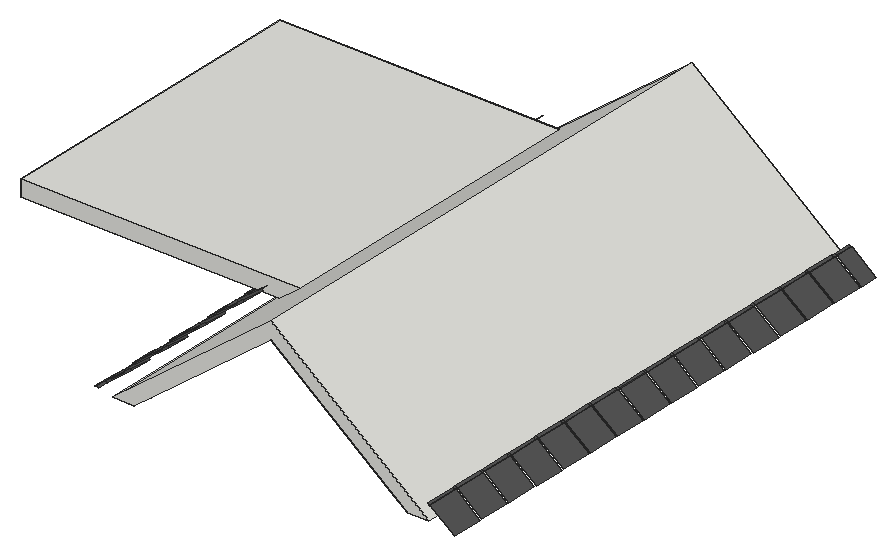
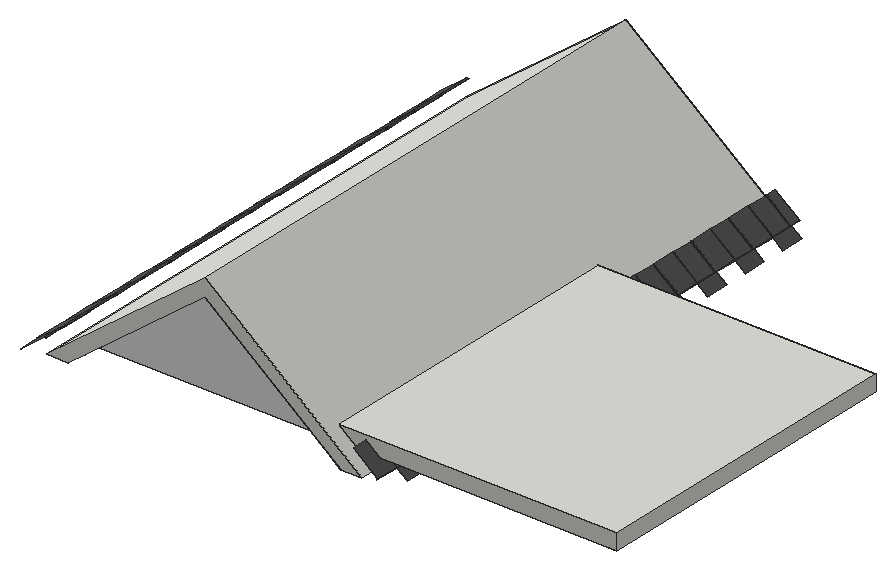
# SketchUp Ruby script. Lengths in inches.
U = 1.inch
M = Sketchup.active_model
def pt(a) = Geom::Point3d.new(a.map { |v| v * U })
def face(e, loops, mat)
  f = e.add_face(loops[0].map { |a| pt(a) })
  loops[1..].each { |l| e.add_face(l.map { |a| pt(a) }).erase! }
  f.material = f.back_material = mat if mat
  f
end
# faces: each face lists its corners as indices into pts; further lists are holes
def faces(e, pts, list, mat = nil) = list.each { |f| face(e, (f[0].is_a?(Array) ? f : [f]).map { |l| l.map { |i| pts[i] } }, mat) }
# xy, xz, yz: faces in a plane at the given z, y or x. An outline is a flat list of corners, or four numbers for a rectangle; further outlines are holes
def ring(l) = l.size == 4 ? [[l[0], l[1]], [l[2], l[1]], [l[2], l[3]], [l[0], l[3]]] : l.each_slice(2).to_a
def flat(e, list, mat, &to3) = list.each { |f| face(e, (f[0].is_a?(Array) ? f : [f]).map { |l| ring(l).map { |u, v| to3.(u, v) } }, mat) }
def xy(e, z, list, mat = nil) = flat(e, list, mat) { |x, y| [x, y, z] }
def xz(e, y, list, mat = nil) = flat(e, list, mat) { |x, z| [x, y, z] }
def yz(e, x, list, mat = nil) = flat(e, list, mat) { |y, z| [x, y, z] }
def lines(e, pts, list) = list.each { |a, b| e.add_line(pt(pts[a]), pt(pts[b])) }
# prism: a flat outline (further loops are holes) pulled along v
def prism(e, loops, v, mat = nil)
  f = face(e, loops, mat); d = Geom::Vector3d.new(v.map { |x| x * U })
  f.pushpull(f.normal.samedirection?(d) ? d.length : -d.length)
end
def box(e, o, s, mat = nil) = prism(e, [[o, [o[0] + s[0], o[1], o[2]], [o[0] + s[0], o[1] + s[1], o[2]], [o[0], o[1] + s[1], o[2]]]], [0, 0, s[2]], mat)
def at(x, y, z, deg = 0) = Geom::Transformation.translation(pt([x, y, z])) * Geom::Transformation.rotation(ORIGIN, Z_AXIS, deg.degrees)
def axes(o, x, y, z) = Geom::Transformation.new([*x, 0, *y, 0, *z, 0, *pt(o).to_a, 1])
def part(name) = M.definitions.add(name)
# library, detail: a bought-in or finely detailed component or shape, given as its bounding box
def library(name, o, s) = part(name).tap { |d| box(d.entities, o, s) }
def detail(e, o, s) = box(e.add_group.entities, o, s)
def put(e, d, t, mat = nil) = e.add_instance(d, t).tap { |i| i.material = mat if mat }
def group(e, t, mat = nil) = e.add_group.tap { |g| g.transformation = t; g.material = mat if mat }.entities
root = M.entities
M.materials.add("[Color M01]").color = [226, 226, 226]
M.materials.add("[Color M06]").color = [86, 86, 86]
xz(root,145.1875,[[245.03,334.59,244.23,335.61,263.13,350.4,263.4375,350.01,263.93,349.38]],"[Color M06]")
xz(root,163.1875,[[245.03,334.59,263.93,349.38,263.4375,350.01,263.13,350.4,244.23,335.61]],"[Color M06]")
xz(root,181.1875,[[245.03,334.59,244.54,335.22,244.23,335.61,263.13,350.4,263.4375,350.01,263.93,349.38]],"[Color M06]")
xz(root,199.1875,[[245.03,334.59,263.93,349.38,263.4375,350.01,263.13,350.4,244.23,335.61,244.54,335.22]],"[Color M06]")
xz(root,217.1875,[[245.03,334.59,244.54,335.22,244.23,335.61,263.13,350.4,263.4375,350.01,263.93,349.38]],"[Color M06]")
xz(root,235.1875,[[245.03,334.59,263.93,349.38,263.4375,350.01,263.13,350.4,244.23,335.61,244.54,335.22]],"[Color M06]")
xz(root,253.1875,[[245.03,334.59,244.23,335.61,263.13,350.4,263.4375,350.01,263.93,349.38]],"[Color M06]")
xz(root,271.1875,[[245.03,334.59,263.93,349.38,263.4375,350.01,263.13,350.4,244.23,335.61]],"[Color M06]")
xz(root,289.1875,[[245.03,334.59,244.54,335.22,244.23,335.61,263.13,350.4,263.4375,350.01,263.93,349.38]],"[Color M06]")
xz(root,307.1875,[[245.03,334.59,263.93,349.38,263.4375,350.01,263.13,350.4,244.23,335.61,244.54,335.22]],"[Color M06]")
xz(root,325.1875,[[245.03,334.59,244.54,335.22,244.23,335.61,263.13,350.4,263.4375,350.01,263.93,349.38]],"[Color M06]")
xz(root,343.1875,[[245.03,334.59,263.93,349.38,263.4375,350.01,263.13,350.4,244.23,335.61,244.54,335.22]],"[Color M06]")
xz(root,361.1875,[[245.03,334.59,244.54,335.22,244.23,335.61,263.13,350.4,263.4375,350.01,263.93,349.38]],"[Color M06]")
xz(root,379.1875,[[245.03,334.59,263.93,349.38,263.4375,350.01,263.13,350.4,244.23,335.61,244.54,335.22]],"[Color M06]")
xz(root,397.1875,[[245.03,334.59,244.23,335.61,263.13,350.4,263.4375,350.01,263.93,349.38]],"[Color M06]")
xz(root,415.1875,[[245.03,334.59,263.93,349.38,263.4375,350.01,263.13,350.4,244.23,335.61]],"[Color M06]")
xz(root,433.1875,[[245.03,334.59,244.23,335.61,263.13,350.4,263.4375,350.01,263.93,349.38]],"[Color M06]")
xz(root,451.1875,[[245.03,334.59,263.93,349.38,263.4375,350.01,263.13,350.4,244.23,335.61]],"[Color M06]")
xz(root,469.1875,[[245.03,334.59,244.54,335.22,244.23,335.61,263.13,350.4,263.4375,350.01,263.93,349.38]],"[Color M06]")
xz(root,487.1875,[[245.03,334.59,263.93,349.38,263.4375,350.01,263.13,350.4,244.23,335.61,244.54,335.22]],"[Color M06]")
xz(root,505.1875,[[245.03,334.59,244.54,335.22,244.23,335.61,263.13,350.4,263.4375,350.01,263.93,349.38]],"[Color M06]")
xz(root,523.1875,[[245.03,334.59,263.93,349.38,263.4375,350.01,263.08,350.46,244.18,335.67,244.23,335.61,244.54,335.22]],"[Color M06]")
p = [[518.42,161.375,328.98],[499.52,161.375,343.77],[499.52,137.375,343.77],[518.42,137.375,328.98],[518.42,187.375,328.98],[499.52,187.375,343.77],
  [499.52,163.375,343.77],[518.42,163.375,328.98],[518.42,213.375,328.98],[499.52,213.375,343.77],[499.52,189.375,343.77],[518.42,189.375,328.98],
  [518.42,239.375,328.98],[499.52,239.375,343.77],[499.52,215.375,343.77],[518.42,215.375,328.98],[518.42,265.375,328.98],[499.52,265.375,343.77],
  [499.52,241.375,343.77],[518.42,241.375,328.98],[518.42,291.375,328.98],[499.52,291.375,343.77],[499.52,267.375,343.77],[518.42,267.375,328.98],
  [518.42,317.375,328.98],[499.52,317.375,343.77],[499.52,293.375,343.77],[518.42,293.375,328.98],[518.42,343.375,328.98],[499.52,343.375,343.77],
  [499.52,319.375,343.77],[518.42,319.375,328.98],[518.42,369.375,328.98],[499.52,369.375,343.77],[499.52,345.375,343.77],[518.42,345.375,328.98],
  [518.42,395.375,328.98],[499.52,395.375,343.77],[499.52,371.375,343.77],[518.42,371.375,328.98],[518.42,421.375,328.98],[499.52,421.375,343.77],
  [499.52,397.375,343.77],[518.42,397.375,328.98],[518.42,447.375,328.98],[499.52,447.375,343.77],[499.52,423.375,343.77],[518.42,423.375,328.98],
  [518.42,473.375,328.98],[499.52,473.375,343.77],[499.52,449.375,343.77],[518.42,449.375,328.98],[518.42,499.375,328.98],[499.52,499.375,343.77],
  [499.52,475.375,343.77],[518.42,475.375,328.98],[518.42,525.375,328.98],[499.52,525.375,343.77],[499.52,501.375,343.77],[518.42,501.375,328.98],
  [518.42,541.1875,328.98],[499.52,541.1875,343.77],[499.52,527.375,343.77],[518.42,527.375,328.98],[236.06,145.1875,329.21],[244.23,145.1875,335.61],
  [244.23,163.1875,335.61],[236.06,163.1875,329.21],[236.06,181.1875,329.21],[244.23,181.1875,335.61],[244.23,199.1875,335.61],[236.06,199.1875,329.21],
  [236.06,217.1875,329.21],[244.23,217.1875,335.61],[244.23,235.1875,335.61],[236.06,235.1875,329.21],[236.06,253.1875,329.21],[244.23,253.1875,335.61],
  [244.23,271.1875,335.61],[236.06,271.1875,329.21],[236.06,289.1875,329.21],[244.23,289.1875,335.61],[244.23,307.1875,335.61],[236.06,307.1875,329.21],
  [236.06,325.1875,329.21],[244.23,325.1875,335.61],[244.23,343.1875,335.61],[236.06,343.1875,329.21],[236.06,361.1875,329.21],[244.23,361.1875,335.61],
  [244.23,379.1875,335.61],[236.06,379.1875,329.21],[236.06,397.1875,329.21],[244.23,397.1875,335.61],[244.23,415.1875,335.61],[236.06,415.1875,329.21],
  [236.06,433.1875,329.21],[244.23,433.1875,335.61],[244.23,451.1875,335.61],[236.06,451.1875,329.21],[236.06,469.1875,329.21],[244.23,469.1875,335.61],
  [244.23,487.1875,335.61],[236.06,487.1875,329.21],[236.06,505.1875,329.21],[244.23,505.1875,335.61],[244.23,523.1875,335.61],[236.06,523.1875,329.21],
  [245.03,145.1875,334.59],[245.03,137.375,334.59],[244.23,137.375,335.61],[245.03,163.1875,334.59],[263.93,145.1875,349.38],[263.93,163.1875,349.38],
  [245.03,181.1875,334.59],[244.54,181.1875,335.22],[245.03,199.1875,334.59],[244.54,199.1875,335.22],[263.93,181.1875,349.38],[263.93,199.1875,349.38],
  [245.03,217.1875,334.59],[244.54,217.1875,335.22],[245.03,235.1875,334.59],[244.54,235.1875,335.22],[263.93,217.1875,349.38],[263.93,235.1875,349.38],
  [245.03,253.1875,334.59],[245.03,271.1875,334.59],[263.93,253.1875,349.38],[263.93,271.1875,349.38],[245.03,289.1875,334.59],[244.54,289.1875,335.22],
  [245.03,307.1875,334.59],[244.54,307.1875,335.22],[263.93,289.1875,349.38],[263.93,307.1875,349.38],[245.03,325.1875,334.59],[244.54,325.1875,335.22],
  [245.03,343.1875,334.59],[244.54,343.1875,335.22],[263.93,325.1875,349.38],[263.93,343.1875,349.38],[245.03,361.1875,334.59],[244.54,361.1875,335.22],
  [245.03,379.1875,334.59],[244.54,379.1875,335.22],[263.93,361.1875,349.38],[263.93,379.1875,349.38],[245.03,397.1875,334.59],[245.03,415.1875,334.59],
  [263.93,397.1875,349.38],[263.93,415.1875,349.38],[245.03,433.1875,334.59],[245.03,451.1875,334.59],[263.93,433.1875,349.38],[263.93,451.1875,349.38],
  [245.03,469.1875,334.59],[244.54,469.1875,335.22],[245.03,487.1875,334.59],[244.54,487.1875,335.22],[263.93,469.1875,349.38],[263.93,487.1875,349.38],
  [245.03,505.1875,334.59],[244.54,505.1875,335.22],[245.03,523.1875,334.59],[244.54,523.1875,335.22],[263.93,505.1875,349.38],[263.93,523.1875,349.38],
  [245.03,541.1875,334.59],[244.18,523.1875,335.67],[244.18,541.1875,335.67],[263.13,137.375,350.4],[263.13,145.1875,350.4],[263.13,163.1875,350.4],
  [263.13,181.1875,350.4],[263.13,199.1875,350.4],[263.13,217.1875,350.4],[263.13,235.1875,350.4],[263.13,253.1875,350.4],[263.13,271.1875,350.4],
  [263.13,289.1875,350.4],[263.13,307.1875,350.4],[263.13,325.1875,350.4],[263.13,343.1875,350.4],[263.13,361.1875,350.4],[263.13,379.1875,350.4],
  [263.13,397.1875,350.4],[263.13,415.1875,350.4],[263.13,433.1875,350.4],[263.13,451.1875,350.4],[263.13,469.1875,350.4],[263.13,487.1875,350.4],
  [263.13,505.1875,350.4],[263.08,523.1875,350.46],[263.08,541.1875,350.46],[497.33,137.375,344.21],[498.91,137.375,342.98],[498.91,161.375,342.98],
  [497.33,161.375,344.21],[498.91,163.375,342.98],[497.33,163.375,344.21],[498.91,187.375,342.98],[497.33,187.375,344.21],[498.91,189.375,342.98],
  [497.33,189.375,344.21],[498.91,213.375,342.98],[497.33,213.375,344.21],[498.91,215.375,342.98],[497.33,215.375,344.21],[498.91,239.375,342.98],
  [497.33,239.375,344.21],[498.91,241.375,342.98],[497.33,241.375,344.21],[498.91,265.375,342.98],[497.33,265.375,344.21],[498.91,267.375,342.98],
  [497.33,267.375,344.21],[498.91,291.375,342.98],[497.33,291.375,344.21],[498.91,293.375,342.98],[497.33,293.375,344.21],[498.91,317.375,342.98],
  [497.33,317.375,344.21],[498.91,319.375,342.98],[497.33,319.375,344.21],[498.91,343.375,342.98],[497.33,343.375,344.21],[498.91,345.375,342.98],
  [497.33,345.375,344.21],[498.91,369.375,342.98],[497.33,369.375,344.21],[498.91,371.375,342.98],[497.33,371.375,344.21],[498.91,395.375,342.98],
  [497.33,395.375,344.21],[498.91,397.375,342.98],[497.33,397.375,344.21],[498.91,421.375,342.98],[497.33,421.375,344.21],[498.91,423.375,342.98],
  [497.33,423.375,344.21],[498.91,447.375,342.98],[497.33,447.375,344.21],[498.91,449.375,342.98],[497.33,449.375,344.21],[498.91,473.375,342.98],
  [497.33,473.375,344.21],[498.91,475.375,342.98],[497.33,475.375,344.21],[498.91,499.375,342.98],[497.33,499.375,344.21],[498.91,501.375,342.98],
  [497.33,501.375,344.21],[498.91,525.375,342.98],[497.33,525.375,344.21],[498.91,527.375,342.98],[497.33,527.375,344.21],[498.91,541.1875,342.98],
  [497.33,541.1875,344.21]]
faces(root,p,[[0,1,2,3],[4,5,6,7],[8,9,10,11],[12,13,14,15],[16,17,18,19],[20,21,22,23],[24,25,26,27],[28,29,30,31],
  [32,33,34,35],[36,37,38,39],[40,41,42,43],[44,45,46,47],[48,49,50,51],[52,53,54,55],[56,57,58,59],[60,61,62,63],
  [64,65,66,67],[68,69,70,71],[72,73,74,75],[76,77,78,79],[80,81,82,83],[84,85,86,87],[88,89,90,91],[92,93,94,95],
  [96,97,98,99],[100,101,102,103],[104,105,106,107],[108,109,110,65],[108,111,66,65],[108,112,113,111],[114,111,66,69,115],[114,116,117,70,69,115],
  [114,118,119,116],[120,116,117,70,73,121],[120,122,123,74,73,121],[120,124,125,122],[126,122,123,74,77],[126,127,78,77],[126,128,129,127],[130,127,78,81,131],
  [130,132,133,82,81,131],[130,134,135,132],[136,132,133,82,85,137],[136,138,139,86,85,137],[136,140,141,138],[142,138,139,86,89,143],[142,144,145,90,89,143],[142,146,147,144],
  [148,144,145,90,93],[148,149,94,93],[148,150,151,149],[152,149,94,97],[152,153,98,97],[152,154,155,153],[156,153,98,101,157],[156,158,159,102,101,157],
  [156,160,161,158],[162,158,159,102,105,163],[162,164,165,106,105,163],[162,166,167,164],[168,164,165,106,169,170],[110,171,172,65],[66,173,174,69],[70,175,176,73],
  [74,177,178,77],[78,179,180,81],[82,181,182,85],[86,183,184,89],[90,185,186,93],[94,187,188,97],[98,189,190,101],[102,191,192,105],
  [169,193,194,170],[195,196,197,198],[197,196,2,1],[199,200,198,197],[201,202,200,199],[201,199,6,5],[202,201,203,204],[205,206,204,203],
  [205,203,10,9],[206,205,207,208],[209,210,208,207],[209,207,14,13],[211,212,210,209],[213,214,212,211],[213,211,18,17],[215,216,214,213],
  [216,215,217,218],[217,215,22,21],[219,220,218,217],[221,222,220,219],[221,219,26,25],[223,224,222,221],[225,226,224,223],[225,223,30,29],
  [227,228,226,225],[229,230,228,227],[229,227,34,33],[230,229,231,232],[233,234,232,231],[233,231,38,37],[234,233,235,236],[236,235,237,238],
  [237,235,42,41],[238,237,239,240],[240,239,241,242],[241,239,46,45],[243,244,242,241],[244,243,245,246],[245,243,50,49],[246,245,247,248],
  [248,247,249,250],[249,247,54,53],[250,249,251,252],[252,251,253,254],[253,251,58,57],[254,253,255,256],[257,258,256,255],[257,255,62,61]],"[Color M06]")
g1 = group(root,at(256.33,157.375,332))
prism(g1,[[[225.78,-20,0],[242.01,-20,0],[121,-20,94.7],[0,-20,0],[16.23,-20,0],[29,-20,10],[121,-20,82],[213,-20,10]]],[0,403.8125,0])
g2 = group(root,at(82.83,292.375,342))
box(g2,[-12,-12,0],[223.5,248.8125,12])
g3 = group(root,at(285.33,520.1875,342),"[Color M01]")
prism(g3,[[[92,9,72],[184,9,0],[0,9,0]]],[0,-9,0])
